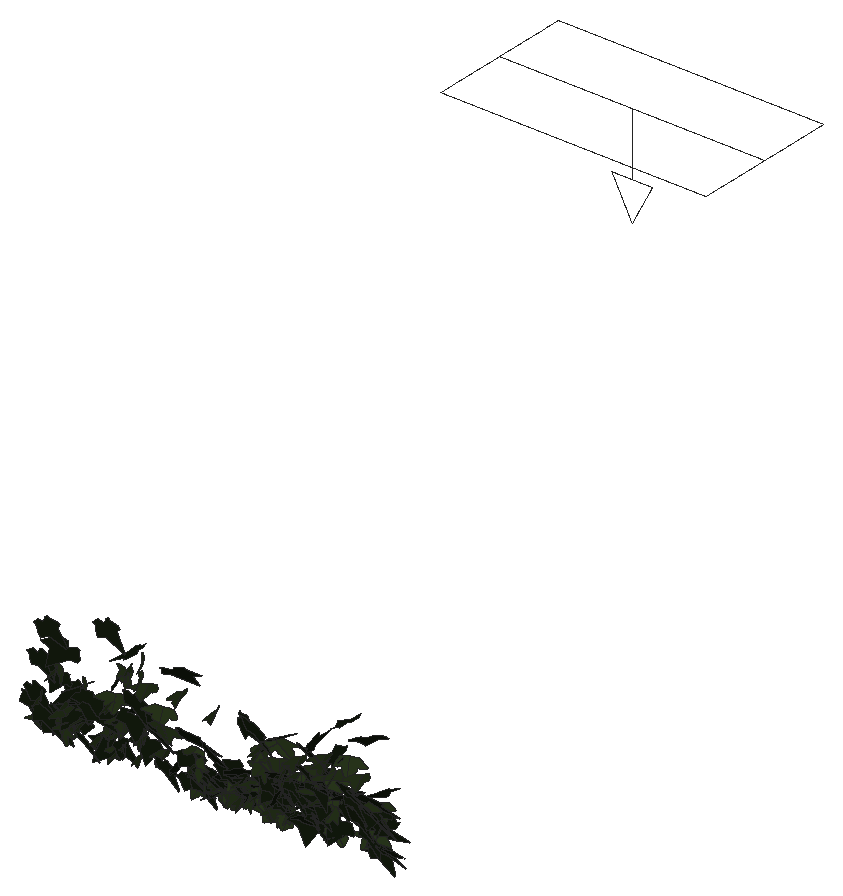
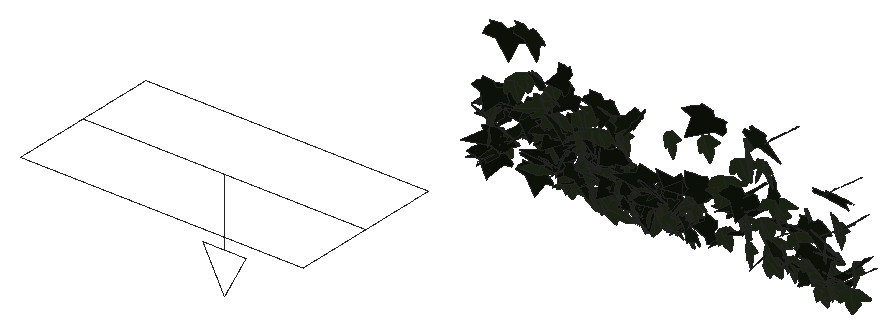
# SketchUp Ruby script. Lengths in millimetres.
U = 1.mm
M = Sketchup.active_model
def pt(a) = Geom::Point3d.new(a.map { |v| v * U })
def face(e, loops, mat)
  f = e.add_face(loops[0].map { |a| pt(a) })
  loops[1..].each { |l| e.add_face(l.map { |a| pt(a) }).erase! }
  f.material = f.back_material = mat if mat
  f
end
# faces: each face lists its corners as indices into pts; further lists are holes
def faces(e, pts, list, mat = nil) = list.each { |f| face(e, (f[0].is_a?(Array) ? f : [f]).map { |l| l.map { |i| pts[i] } }, mat) }
# xy, xz, yz: faces in a plane at the given z, y or x. An outline is a flat list of corners, or four numbers for a rectangle; further outlines are holes
def ring(l) = l.size == 4 ? [[l[0], l[1]], [l[2], l[1]], [l[2], l[3]], [l[0], l[3]]] : l.each_slice(2).to_a
def flat(e, list, mat, &to3) = list.each { |f| face(e, (f[0].is_a?(Array) ? f : [f]).map { |l| ring(l).map { |u, v| to3.(u, v) } }, mat) }
def xy(e, z, list, mat = nil) = flat(e, list, mat) { |x, y| [x, y, z] }
def xz(e, y, list, mat = nil) = flat(e, list, mat) { |x, z| [x, y, z] }
def yz(e, x, list, mat = nil) = flat(e, list, mat) { |y, z| [x, y, z] }
def lines(e, pts, list) = list.each { |a, b| e.add_line(pt(pts[a]), pt(pts[b])) }
# prism: a flat outline (further loops are holes) pulled along v
def prism(e, loops, v, mat = nil)
  f = face(e, loops, mat); d = Geom::Vector3d.new(v.map { |x| x * U })
  f.pushpull(f.normal.samedirection?(d) ? d.length : -d.length)
end
def box(e, o, s, mat = nil) = prism(e, [[o, [o[0] + s[0], o[1], o[2]], [o[0] + s[0], o[1] + s[1], o[2]], [o[0], o[1] + s[1], o[2]]]], [0, 0, s[2]], mat)
def at(x, y, z, deg = 0) = Geom::Transformation.translation(pt([x, y, z])) * Geom::Transformation.rotation(ORIGIN, Z_AXIS, deg.degrees)
def axes(o, x, y, z) = Geom::Transformation.new([*x, 0, *y, 0, *z, 0, *pt(o).to_a, 1])
def part(name) = M.definitions.add(name)
# library, detail: a bought-in or finely detailed component or shape, given as its bounding box
def library(name, o, s) = part(name).tap { |d| box(d.entities, o, s) }
def detail(e, o, s) = box(e.add_group.entities, o, s)
def put(e, d, t, mat = nil) = e.add_instance(d, t).tap { |i| i.material = mat if mat }
def group(e, t, mat = nil) = e.add_group.tap { |g| g.transformation = t; g.material = mat if mat }.entities
root = M.entities
M.materials.add("efeu1").color = [18, 25, 13]
M.materials.add("efeu2").color = [43, 57, 29]
c1 = part("ivyleaf_10")
p = [[0,12.8,-0.8],[-1.5,51.3,-10.9],[-4.9,51,-11.6],[-13.6,26.5,-7.3],[-13.2,15.9,-4.6],[-21.1,19.3,-7.2],
  [-29.5,16.3,-8.3],[-29.2,8.3,-6.2],[-19.7,-9.8,0.5],[-7.6,-13,4],[1,-12.2,5.8],[-0.4,51.1,-11.1],
  [-1.5,51.1,-10.9],[1,-12.4,5.9],[16.9,-12.4,3.5],[35.1,9.1,-5.1],[35,12.9,-6.1],[20.5,16.4,-4.9],
  [15.8,15,-3.8],[15.3,27.6,-7.1],[12.8,31.3,-7.8]]
faces(c1.entities,p,[[0,1,2,3,4,5,6,7,8,9,10],[11,12,0,13,14,15,16,17,18,19,20]],"efeu2")
c2 = part("ivyleaf_9")
p = [[39.1,54.8,31.7],[34.5,51.8,30.2],[-5.3,25.2,17.3],[-17.9,28.3,20.9],[-21.6,21.7,17],[-20.2,4.3,5.3],
  [-22.9,-0.3,2.5],[-17.1,-4,-0.6],[-2,-2.1,-1.2],[-0.7,-15.4,-10.1],[16.6,-22.3,-16.7],[21.1,-15.1,-12.5],
  [32.7,-10.7,-11],[46.1,-1.8,-6.6],[30.8,11.2,3.8]]
faces(c2.entities,p,[[0,1,2,3,4,5,6,7,8,9,10,11,12,13,14]],"efeu1")
c3 = part("Group240\#1")
p = [[0,0,0],[0,0,-197.7],[-63.2,0,-197.7],[411.6,-228.5,0],[-411.6,-228.5,0],[411.6,228.5,0],
  [411.6,0,0],[-411.6,228.5,0],[63.2,0,-197.7],[-411.6,0,0],[0,0,-320]]
lines(c3.entities,p,[[0,1],[1,2],[3,4],[5,6],[7,5],[1,8],[9,0],[0,6],[8,10],[4,9],[6,3],[2,10],
  [9,7]])
c4 = part("Rectangle Light\#2")
put(c4.entities,c3,at(0,0,0))
put(root,c1,axes([2467.9,943.6,1872.4],[-0.26486,-0.88516,0.00004],[-0.00622,0.00047,-0.89602],[1.68462,-0.13916,-0.0033]))
put(root,c1,axes([2705.5,950.2,1793.7],[0.91031,-0.25372,0.7536],[1.32752,-0.28837,-0.53979],[0.7266,0.84471,0.04208]))
put(root,c1,axes([2420.8,938.9,1761.7],[-1.66373,0.07531,0.0181],[-0.0341,0.00288,-0.87741],[-0.14341,-0.87436,-0.00133]))
put(root,c2,axes([2316.7,953.3,1750.5],[-0.39409,-0.85297,0.01207],[0.00655,-0.01326,-0.87772],[1.62353,-0.20699,0.00647]))
put(root,c1,axes([2361.1,945.6,1853.5],[-0.87128,-0.74486,0.14939],[-0.04243,-0.16117,-0.87192],[1.44522,-0.45378,0.06446]))
put(root,c2,axes([3038.7,936,1785.1],[1.61238,-0.09249,0.25483],[0.49062,0.01608,-0.85118],[0.15967,0.88454,0.04212]))
put(root,c1,axes([2910.3,944.7,1850.7],[-0.6012,-0.83319,0.06967],[0.02337,-0.07909,-0.89019],[1.59108,-0.31366,0.0394]))
put(root,c1,axes([2344,947.8,1718],[0.72212,-0.75077,0.22454],[0.4013,-0.14246,-0.83264],[1.43639,0.41724,0.11974]))
put(root,c1,axes([2796.7,947.1,1765.9],[0.88227,-0.70071,0.2164],[0.46375,-0.09429,-0.82731],[1.31643,0.50283,0.14642]))
put(root,c1,axes([2682.9,937.4,1657.3],[0.9527,-0.56773,-0.41231],[-0.3179,0.3955,-0.74738],[1.297,0.51396,0.11967]))
put(root,c2,axes([2330.5,942,1942.5],[-0.88006,0.71726,-0.27291],[0.03704,-0.30756,-0.84131],[-1.46009,-0.44013,0.14315]))
put(root,c1,axes([2261.2,947,1788.5],[-1.27395,-0.57202,0.12507],[0.12482,-0.26201,-0.84733],[1.10738,-0.62853,0.23939]))
put(root,c1,axes([3023,946,1834],[-0.68727,-0.80854,0.10452],[0.03048,-0.12133,-0.88322],[1.55132,-0.35582,0.06366]))
put(root,c2,axes([2679.9,953.4,1854.5],[0.65585,-0.85266,0.25567],[0.23139,-0.2265,-0.91927],[1.67828,0.36444,0.02683]))
put(root,c2,axes([3057.5,948.2,1747.2],[1.01963,-0.67289,0.13481],[0.14364,-0.11221,-0.86005],[1.29817,0.54093,-0.01072]))
put(root,c2,axes([2190,941.3,1740.7],[0.65041,-0.70724,-0.41439],[0.11605,0.46966,-0.75127],[1.55573,0.26064,0.22929]))
put(root,c2,axes([2769.1,930,1680.7],[0.1576,-0.22127,0.85612],[0.86263,0.74893,0.14972],[-1.445,0.42296,0.18276]))
put(root,c1,axes([2710.1,946,1801.6],[0.01408,-0.89116,0.03833],[-0.00107,-0.03834,-0.89119],[1.69763,0.00736,-0.00088]))
put(root,c2,axes([2231.7,945.4,1980.4],[0.44976,-0.80397,-0.30337],[-0.05454,0.30709,-0.83613],[1.63451,0.23147,0.05557]))
put(root,c2,axes([2549.8,939.8,1678],[1.3016,-0.47552,-0.21419],[-0.21038,0.21303,-0.8259],[0.97003,0.68426,0.10828]))
put(root,c2,axes([2756.8,959.4,1711.9],[-1.13486,-0.57406,0.25472],[0.02832,-0.36406,-0.78564],[1.19494,-0.53657,0.26053]))
put(root,c2,axes([2776.3,929,1862.9],[0.53766,0.81104,0.16092],[-0.04042,0.17712,-0.85538],[-1.57315,0.27264,0.07698]))
put(root,c2,axes([2596.5,941.1,1650.7],[-0.70916,0.74438,-0.22777],[0.13305,-0.2195,-0.83171],[-1.47555,-0.37755,0.03448]))
put(root,c2,axes([2817.1,952.6,1730],[0.17226,-0.85614,-0.00431],[-0.02833,0.00276,-0.86079],[1.62917,0.09057,-0.01451]))
put(root,c1,axes([2938.2,944.8,1811.7],[0.50976,-0.85015,-0.09039],[-0.00673,0.09362,-0.89101],[1.62712,0.26673,0.02463]))
put(root,c2,axes([2004.4,954.7,1693.1],[-0.03885,-0.85712,0.0673],[0.01629,-0.06752,-0.8573],[1.63621,-0.01968,0.01013]))
put(root,c2,axes([3004.6,952.1,1769],[0.19705,-0.87319,-0.05486],[0.00113,0.05531,-0.87928],[1.66514,0.1033,0.00709]))
put(root,c2,axes([2819.9,955.3,1756],[-0.70981,-0.79026,-0.03407],[0.06483,0.02158,-0.87358],[1.50402,-0.37389,0.02158]))
put(root,c1,axes([2780.2,943,1777.8],[0.86751,-0.73664,-0.18739],[-0.00785,0.2161,-0.85954],[1.44661,0.44293,0.10771]))
put(root,c1,axes([2109.7,939.1,1699.3],[-0.69981,-0.72469,-0.32601],[0.24848,0.29924,-0.81244],[1.49181,-0.3898,-0.01761]))
put(root,c2,axes([2048.8,947.2,1678.2],[-0.01924,-0.79231,-0.36591],[0.01801,0.36581,-0.79236],[1.66087,-0.01315,0.00435]))
put(root,c1,axes([2094.2,943.9,1646.4],[-1.33967,0.42463,-0.15601],[0.15741,-0.16289,-0.81655],[-0.84645,-0.70234,0.09506]))
put(root,c2,axes([2822.5,952.6,1746.8],[-0.02178,-0.87439,-0.09647],[-0.00803,0.09654,-0.87445],[1.67422,-0.01091,-0.00545]))
put(root,c2,axes([2107.4,953.8,1869.4],[-1.59187,-0.22783,-0.10408],[0.23043,-0.05016,-0.86323],[0.41731,-0.84138,0.07964]))
put(root,c1,axes([2353.6,946.1,1709.7],[0.03956,-0.8764,-0.02765],[-0.00239,0.02762,-0.87664],[1.66879,0.02082,-0.0006]))
put(root,c2,axes([2761.6,939.2,1748],[1.11776,-0.20498,0.58914],[1.17354,0.06847,-0.59087],[0.17944,0.82905,0.19446]))
put(root,c1,axes([2507.7,948,1683.9],[0.21064,-0.85815,0.05755],[0.02757,-0.05616,-0.86523],[1.63668,0.11139,0.00717]))
put(root,c2,axes([2498.8,940,1658.9],[0.41772,-0.58169,-0.59289],[0.01772,0.61492,-0.59986],[1.58068,0.14683,0.16341]))
put(root,c2,axes([3059.5,954.3,1764.8],[-1.26539,-0.50789,-0.24826],[0.46841,0.08498,-0.83298],[0.9686,-0.70461,0.07849]))
put(root,c2,axes([2884.2,925.3,1878.6],[0.2539,0.24727,0.91679],[0.89394,0.78742,-0.28073],[-1.57061,0.48815,-0.01157]))
put(root,c2,axes([2151.7,956.6,1635.3],[0.54439,-0.70731,0.40705],[0.27908,-0.37976,-0.76294],[1.52787,0.32139,-0.00567]))
put(root,c2,axes([2861.5,939.6,1853.5],[1.65475,-0.26156,-0.28108],[-0.51333,0.07912,-0.90794],[0.52006,0.91033,-0.00185]))
put(root,c1,axes([2737.8,942.1,1662.1],[-1.53367,0.31222,-0.04686],[0.08019,-0.02096,-0.8642],[-0.5955,-0.80693,0.00432]))
put(root,c2,axes([2022.3,950.1,1822.5],[0.45856,-0.83446,-0.16753],[-0.0346,0.16902,-0.86806],[1.61946,0.23989,0.02889]))
put(root,c2,axes([2193.8,956.4,1755.8],[-1.03123,-0.66738,-0.09407],[0.21794,0.02778,-0.85671],[1.26407,-0.54924,0.07097]))
put(root,c2,axes([2313.7,954.3,1803.7],[0.31449,-0.85872,0.01341],[-0.00061,-0.01372,-0.87447],[1.63451,0.16522,-0.00291]))
put(root,c2,axes([2363.2,951.9,1744.3],[0.9242,-0.70894,0.17463],[0.24251,-0.12422,-0.85862],[1.36826,0.50087,0.03423]))
put(root,c2,axes([2490.1,948.9,1706.7],[0.22463,-0.80548,-0.30843],[0.13705,0.31942,-0.80662],[1.6358,0.08385,0.10994]))
put(root,c2,axes([2594.9,950.3,1704.2],[0.80018,-0.76253,-0.03422],[0.08039,0.06225,-0.86818],[1.45048,0.41721,0.06699]))
put(root,c1,axes([2828.8,948.1,1814.3],[-0.46004,-0.85367,0.03783],[0.01161,-0.04104,-0.88707],[1.62626,-0.24119,0.01704]))
put(root,c2,axes([2701.3,934.4,1723.1],[0.15563,0.84621,0.05009],[-0.16196,0.05826,-0.84536],[-1.60517,0.07617,0.09015]))
put(root,c2,axes([2749.6,932.9,1826.6],[-0.04628,0.84008,0.20504],[-0.03955,0.20449,-0.84031],[-1.6453,-0.02854,0.01443]))
put(root,c1,axes([2712.6,943.5,1749.4],[1.19721,-0.54171,-0.29332],[-0.24451,0.29464,-0.81968],[1.14664,0.62843,0.13147]))
put(root,c1,axes([2913.3,948.2,1833.8],[-0.35011,-0.86827,0.02169],[0.00942,-0.02321,-0.8875],[1.65299,-0.18377,0.00965]))
put(root,c2,axes([2455.1,934.6,1936],[1.53035,0.42348,0.0933],[0.17778,0.02278,-0.90849],[-0.80591,0.80917,-0.02325]))
put(root,c2,axes([2882.3,956.2,1763.7],[0.09573,-0.87118,0.02439],[-0.00125,-0.02447,-0.87263],[1.65867,0.05026,-0.00207]))
put(root,c1,axes([2122.4,947.9,1661.6],[-0.72568,-0.78406,0.03692],[-0.02053,-0.03581,-0.87184],[1.49374,-0.3814,0.00595]))
put(root,c1,axes([2531.9,933.6,1692],[0.25909,-0.56883,-0.73164],[0.61868,0.72182,-0.50071],[1.65173,-0.18114,0.30232]))
put(root,c2,axes([2969,949.6,1787.5],[1.04021,-0.69755,0.00833],[0.15036,0.05138,-0.88119],[1.31913,0.5442,0.09387]))
put(root,c2,axes([2251.7,954.2,1651.2],[-1.58105,-0.14055,-0.11339],[0.21207,0.02113,-0.84254],[0.27048,-0.83817,-0.00222]))
put(root,c1,axes([2813.6,933.5,1696.6],[0.3828,0.06766,-0.86768],[-0.86684,0.76704,-0.04577],[1.41144,0.45273,0.20721]))
put(root,c1,axes([2881.7,951,1744.5],[-0.89868,-0.71255,0.14671],[-0.03727,-0.16239,-0.85174],[1.38406,-0.46703,0.07232]))
put(root,c1,axes([2404.3,954.1,1798.4],[-1.27482,-0.53387,0.18484],[0.12371,-0.35761,-0.79734],[1.0681,-0.59578,0.31296]))
put(root,c2,axes([2404.9,958,1649.7],[0.44725,-0.80998,0.18846],[0.10699,-0.17992,-0.84337],[1.57911,0.2416,0.00377]))
put(root,c2,axes([3030,954,1753.1],[0.93049,-0.7024,0.1556],[0.18839,-0.12067,-0.85572],[1.3562,0.49868,0.01211]))
put(root,c2,axes([2248.8,954.4,1745.2],[-1.61597,0.07599,0.12325],[-0.24749,-0.07772,-0.84791],[-0.1212,-0.85445,0.08809]))
put(root,c1,axes([2341.7,944.3,1868.8],[0.36417,-0.81308,-0.32498],[-0.0473,0.32747,-0.83395],[1.66582,0.18705,0.04737]))
put(root,c2,axes([2566.8,940.8,1685.1],[1.33692,-0.35338,-0.35224],[-0.3711,0.36548,-0.75552],[0.8741,0.69566,0.218]))
put(root,c2,axes([2537.4,961.6,1725.9],[0.31583,-0.40279,0.79125],[0.621,-0.72095,-0.43544],[1.57155,0.36583,0.01305]))
put(root,c1,axes([2091.7,944.7,1801.9],[0.86528,-0.68958,-0.30711],[-0.0766,0.33586,-0.81371],[1.43464,0.43384,0.14178]))
put(root,c2,axes([2077.1,964.5,1786],[-0.60418,-0.70125,0.37246],[-0.1548,-0.3703,-0.7665],[1.50324,-0.31998,0.07077]))
put(root,c1,axes([2298.4,940.7,1866.4],[0.73702,-0.53266,-0.59096],[-0.49411,0.53666,-0.65385],[1.43128,0.45956,0.07859]))
put(root,c2,axes([2737.8,954,1720.6],[0.33451,-0.83791,-0.15723],[0.00211,0.16076,-0.85548],[1.62253,0.17254,0.03353]))
put(root,c1,axes([2772,948.8,1788.6],[-1.3717,-0.4905,0.00951],[0.05881,-0.06226,-0.86908],[0.93183,-0.7181,0.06886]))
put(root,c2,axes([2658.5,942.8,1866.2],[0.96672,-0.53668,-0.55848],[-0.66997,0.43494,-0.73813],[1.31307,0.61704,0.03455]))
put(root,c2,axes([2998.9,955.6,1721],[0.70359,-0.78355,0.06825],[0.05768,-0.06116,-0.86639],[1.49579,0.37093,0.00131]))
put(root,c2,axes([2903.3,960.8,1728.6],[-0.84018,-0.74203,-0.00391],[0.09077,-0.02384,-0.86178],[1.40933,-0.44083,0.05318]))
put(root,c1,axes([2931.3,949.7,1708.6],[1.28701,-0.5645,-0.16398],[-0.19921,0.13032,-0.88029],[1.10088,0.68352,0.03241]))
put(root,c1,axes([2246.1,947.2,1764.7],[0.03971,-0.86574,-0.20459],[0.00101,0.20466,-0.86598],[1.69307,0.02018,0.00532]))
put(root,c1,axes([2886.8,942,1678.6],[-0.55208,0.77639,0.22455],[-0.21603,0.19708,-0.82802],[-1.52294,-0.3094,0.03605]))
put(root,c2,axes([3051,938,1956.8],[0.61842,0.83188,-0.10686],[-0.19135,-0.07514,-0.89066],[-1.58473,0.3337,0.06584]))
put(root,c2,axes([2840.1,949.9,1790.3],[1.22609,-0.60844,-0.01915],[0.14418,0.1078,-0.87649],[1.14955,0.63543,0.13035]))
put(root,c2,axes([2043.2,948.9,1917.1],[0.587,-0.72583,-0.40656],[-0.04612,0.42558,-0.77817],[1.58268,0.2816,0.12811]))
put(root,c1,axes([2986,949.9,1865.1],[1.11361,0.65554,-0.11344],[-0.26983,-0.02474,-0.87422],[-1.23708,0.59551,0.08856]))
put(root,c2,axes([2799.1,954.6,1705.5],[-1.53306,0.2288,-0.18474],[0.31242,-0.09712,-0.83604],[-0.46436,-0.8207,0.04743]))
put(root,c2,axes([2973.5,947.4,1734],[0.97047,-0.59501,-0.36846],[-0.39027,0.30886,-0.78254],[1.27351,0.54807,0.04097]))
put(root,c2,axes([2708.8,949.4,1669.3],[0.46911,0.5613,-0.58767],[-0.46184,-0.53525,-0.61302],[-1.47609,0.34585,0.00504]))
put(root,c1,axes([2766.4,944.3,1839.1],[1.29645,0.29451,0.46585],[0.6213,0.38113,-0.7183],[-0.84513,0.73197,0.18657]))
put(root,c1,axes([2170,943.7,1788],[0.43763,-0.69637,-0.47194],[-0.08556,0.47838,-0.72777],[1.59872,0.21622,0.09024]))
put(root,c1,axes([2237.6,949.9,1678.2],[0.73526,-0.74565,-0.13769],[0.17887,0.20043,-0.8217],[1.43198,0.35782,0.17334]))
put(root,c2,axes([2516.2,957,1641.9],[0.47088,-0.81913,-0.07357],[0.0296,0.08147,-0.85483],[1.56497,0.24493,0.0383]))
put(root,c1,axes([2694.9,955.2,1691.8],[1.42292,-0.37077,0.24795],[0.47448,-0.05394,-0.83239],[0.70392,0.78584,0.05985]))
put(root,c1,axes([2613.4,950.7,1636.5],[-1.40709,-0.37225,0.10008],[-0.1704,-0.04472,-0.82775],[0.71355,-0.74473,-0.00032]))
put(root,c1,axes([2821.1,955.1,1765.1],[-0.12246,-0.8658,0.10447],[-0.05796,-0.10246,-0.86789],[1.65872,-0.0675,-0.02261]))
put(root,c1,axes([2904.6,953.8,1783.9],[-0.7516,-0.78033,0.06766],[0.05443,-0.09009,-0.87207],[1.48969,-0.39041,0.066]))
put(root,c1,axes([2515.6,953.7,1630.9],[1.24501,-0.54678,-0.05877],[-0.07865,0.04219,-0.85257],[1.04367,0.65544,0.00585]))
put(root,c1,axes([3077.8,950.7,1770.8],[-1.25736,-0.5489,-0.16054],[0.38831,0.00292,-0.84964],[1.01681,-0.67987,0.12596]))
put(root,c2,axes([2986.9,937.7,1975.5],[0.01006,0.86938,0.22364],[-0.14922,0.22324,-0.86596],[-1.70194,-0.01443,0.07724]))
put(root,c2,axes([2867.7,942.4,1667.5],[0.98909,0.64386,-0.22357],[-0.34715,-0.1395,-0.82577],[-1.24985,0.54828,0.05243]))
put(root,c2,axes([2959.5,949.3,1871.5],[-1.08075,0.67413,-0.07436],[0.06867,-0.06682,-0.88129],[-1.28896,-0.56879,0.01539]))
put(root,c1,axes([2787.8,947,1772.8],[0.20165,-0.78561,-0.3752],[-0.0369,0.37575,-0.79222],[1.65653,0.104,0.02802]))
put(root,c1,axes([2566.3,951.4,1852.2],[-0.05275,-0.87059,-0.14113],[-0.00528,0.14129,-0.871],[1.67852,-0.02691,-0.00718]))
put(root,c1,axes([2284.7,952.9,1729.5],[-0.98379,-0.71114,-0.02205],[0.11719,-0.01756,-0.8771],[1.34901,-0.51708,0.06011]))
put(root,c2,axes([2895.5,943.6,1754.8],[0.99429,0.59745,-0.33857],[-0.59781,-0.1704,-0.78538],[-1.16222,0.59877,0.11432]))
put(root,c2,axes([2137.9,962.5,1702.6],[-1.4103,-0.42406,-0.03234],[0.05068,0.01856,-0.85377],[0.80782,-0.74149,-0.00288]))
put(root,c2,axes([2002.4,954.8,1721.6],[0.66275,-0.76295,-0.24811],[-0.10483,0.2471,-0.83715],[1.52328,0.34895,0.05033]))
put(root,c2,axes([2627.9,940.5,1706.9],[0.80073,-0.02688,0.7568],[1.28025,0.41088,-0.35937],[-0.66192,0.76219,0.22043]))
put(root,c1,axes([2497.2,962.1,1712.1],[0.50292,0.58423,-0.62362],[-0.712,-0.50779,-0.63424],[-1.46222,0.4482,0.09434]))
put(root,c2,axes([2866.2,962.2,1671.4],[0.34879,-0.84035,0.05099],[-0.0033,-0.05256,-0.86001],[1.6023,0.18282,-0.01287]))
put(root,c1,axes([2774.5,950.3,1738.4],[-0.74948,0.77477,0.0623],[-0.36984,-0.03052,-0.84884],[-1.43232,-0.39752,0.18658]))
put(root,c2,axes([2759.6,949,1710.1],[1.59715,-0.16882,0.03563],[0.06069,-0.02215,-0.85586],[0.32271,0.83965,-0.01541]))
put(root,c1,axes([2188.1,958.1,1726.4],[-0.75727,-0.75041,0.18218],[0.02116,-0.21049,-0.84273],[1.46951,-0.38367,0.10602]))
put(root,c1,axes([2262.7,962.2,1637.8],[-0.24892,-0.75175,0.3805],[-0.08078,-0.37869,-0.76276],[1.60153,-0.13594,0.02067]))
put(root,c2,axes([2352.8,967,1689.5],[-0.58891,-0.78496,0.11855],[0.01763,-0.1308,-0.84188],[1.51077,-0.30446,0.05603]))
put(root,c1,axes([2832,954.7,1759.3],[1.48089,0.40461,0.02343],[0.03195,0.01849,-0.87698],[-0.77068,0.77824,0.00866]))
put(root,c2,axes([2846,966.2,1642],[-0.63565,-0.78503,0.02418],[0.05186,-0.03785,-0.85219],[1.49387,-0.33272,0.03988]))
put(root,c1,axes([2642.2,966.2,1684.1],[-0.74241,-0.47484,0.59059],[-0.22658,-0.6176,-0.57518],[1.42435,-0.34574,0.21633]))
put(root,c2,axes([2868.6,957.3,1703.3],[0.46618,-0.78538,-0.25499],[-0.05531,0.2576,-0.82136],[1.57057,0.24219,0.04676]))
put(root,c1,axes([2025,949.2,1703.4],[0.08591,-0.78293,-0.37668],[0.11766,0.37913,-0.78061],[1.64937,0.01374,0.0753]))
put(root,c1,axes([2068.1,953.2,1790.5],[0.07515,-0.84868,-0.1854],[0.06464,0.18696,-0.84858],[1.65204,0.03129,0.04163]))
put(root,c1,axes([2650.4,957.4,1685],[-0.14758,-0.84578,0.03604],[-0.01332,-0.03555,-0.84932],[1.6111,-0.07777,-0.00372]))
put(root,c1,axes([2283.1,958.9,1718.8],[0.9157,-0.71154,0.07292],[0.15214,-0.03383,-0.85765],[1.35276,0.48545,0.0471]))
put(root,c1,axes([2107.9,953.5,1719.8],[0.1026,-0.82425,-0.20479],[0.05404,0.20683,-0.82501],[1.6155,0.04543,0.0406]))
put(root,c1,axes([2900.5,955.8,1723],[-0.40665,-0.8455,-0.05609],[0.04161,0.05233,-0.87204],[1.61216,-0.21462,0.00836]))
put(root,c2,axes([3039.5,965.9,1680.7],[0.15196,-0.84584,0.09159],[-0.01234,-0.0926,-0.84946],[1.61916,0.07868,-0.01507]))
put(root,c1,axes([2208.9,956.5,1654.5],[-0.02567,-0.86483,-0.06485],[0.01894,0.0647,-0.86489],[1.65045,-0.01419,0.00892]))
put(root,c1,axes([2603.8,966.7,1642.2],[-0.2302,-0.68836,0.4772],[0.32357,-0.49229,-0.66703],[1.56091,0.00053,0.20865]))
put(root,c2,axes([2587.3,940.9,1679.9],[1.07226,0.25057,0.59872],[0.91294,0.37331,-0.60762],[-0.8321,0.73248,0.10486]))
put(root,c2,axes([2139.4,959.4,1756.4],[-1.49804,0.32185,-0.13002],[0.21007,-0.07345,-0.84998],[-0.62635,-0.7944,0.02591]))
put(root,c2,axes([2767,959.9,1678.2],[0.34726,-0.80067,-0.25157],[0.0127,0.25883,-0.81891],[1.59723,0.17202,0.06121]))
put(root,c2,axes([2636.9,959.4,1708.9],[-1.51427,0.28436,-0.02191],[0.02531,-0.02785,-0.84465],[-0.54221,-0.79546,0.02175]))
put(root,c1,axes([2805.3,961.5,1712.6],[0.87746,-0.71773,0.13539],[0.20011,-0.09321,-0.85222],[1.37559,0.47139,0.03762]))
put(root,c2,axes([2060,954.9,1652.6],[0.2213,-0.67687,-0.5282],[0.03448,0.53484,-0.68139],[1.63368,0.0804,0.08593]))
put(root,c1,axes([2275.4,954.6,1646.1],[-0.05824,-0.83738,-0.23344],[0.00829,0.23343,-0.83793],[1.65445,-0.03064,-0.00402]))
put(root,c2,axes([2351.7,958.8,1758.4],[0.86776,-0.72125,-0.16298],[0.01203,0.19526,-0.84646],[1.40724,0.44308,0.10773]))
put(root,c2,axes([2870.9,947.1,1683.5],[0.90823,-0.00913,0.77376],[1.43221,0.21722,-0.46156],[-0.34303,0.88275,0.12158]))
put(root,c1,axes([3054.6,960,1676.9],[1.4009,0.34389,-0.30202],[-0.55886,-0.08389,-0.81118],[-0.66815,0.79119,0.04526]))
put(root,c1,axes([2540.8,961.7,1657.1],[-1.13091,-0.60841,0.14157],[0.06333,-0.22595,-0.83135],[1.18718,-0.56752,0.17921]))
put(root,c1,axes([2877.6,956.2,1789.1],[1.21378,-0.52621,-0.27544],[-0.29793,0.24094,-0.82277],[1.09042,0.65158,0.0818]))
put(root,c2,axes([2946.5,965.3,1673.5],[-1.47061,-0.20546,-0.31245],[0.58853,0.05222,-0.7991],[0.40018,-0.83184,0.02701]))
put(root,c2,axes([2464.5,955.6,1755.8],[1.54316,-0.25843,0.35026],[0.64564,-0.08882,-0.85084],[0.51906,0.87877,0.01701]))
put(root,c1,axes([2707.1,964.1,1691],[0.47193,-0.79606,0.19306],[0.27043,-0.15685,-0.82926],[1.53534,0.27232,0.08673]))
put(root,c1,axes([2575.6,962.9,1656.3],[-0.09348,-0.8447,0.12551],[-0.05488,-0.12401,-0.84585],[1.62435,-0.0528,-0.02135]))
put(root,c2,axes([2877,945.7,1762.3],[1.34216,0.52338,0.11083],[0.15554,0.07583,-0.87812],[-1.00623,0.70983,0.01209]))
put(root,c1,axes([2330.3,956.9,1645.6],[0.14724,-0.82771,-0.20258],[0.07415,0.20663,-0.8294],[1.62009,0.06577,0.05637]))
put(root,c1,axes([2643.9,962.6,1633.9],[0.04653,-0.84633,0.0904],[0.02318,-0.09008,-0.84663],[1.61974,0.0256,0.00952]))
put(root,c1,axes([2341,952.3,1914.2],[0.3119,-0.73005,-0.46171],[-0.07433,0.4632,-0.74628],[1.6423,0.15962,0.05391]))
put(root,c2,axes([2975.4,947.1,1765.8],[0.45263,0.83183,0.02298],[-0.0045,0.02458,-0.86511],[-1.58374,0.23766,0.00903]))
put(root,c1,axes([2687.7,961.6,1693.5],[-0.64019,-0.78053,0.07618],[-0.03743,-0.07447,-0.84985],[1.4921,-0.33676,0.01137]))
put(root,c1,axes([2251.3,960.2,1688.3],[-0.60999,-0.80189,-0.0093],[0.00138,0.00973,-0.86356],[1.52626,-0.32049,-0.00293]))
put(root,c1,axes([2940.5,942.7,1795],[0.02325,-0.03147,0.96719],[0.63208,0.90866,0.02537],[-1.72987,0.33159,0.02227]))
put(root,c1,axes([2817.3,954.1,1726.9],[-0.63088,0.80212,0.11016],[-0.10997,0.09529,-0.86775],[-1.53699,-0.33606,0.01687]))
put(root,c1,axes([2496.4,955.3,1699],[1.07537,-0.5662,-0.32944],[-0.16746,0.36552,-0.77912],[1.23542,0.54239,0.18115]))
put(root,c1,axes([2923.9,960.4,1729.2],[1.37542,0.46259,-0.0301],[-0.05157,-0.01349,-0.85806],[-0.88076,0.72319,0.00324]))
put(root,c2,axes([3107.2,949.6,1719.1],[-0.59763,0.55915,0.59705],[-0.77323,0.44846,-0.63367],[-1.35121,-0.50394,0.09855]))
put(root,c1,axes([2623.7,962.3,1636.6],[-1.06687,-0.6392,0.08068],[0.05206,-0.13046,-0.84354],[1.22508,-0.55111,0.1061]))
put(root,c1,axes([2303.2,943.1,1862.8],[-0.02006,0.17131,0.86807],[-0.69357,0.79024,-0.16038],[-1.53451,-0.35941,0.06114]))
put(root,c1,axes([2143.3,963.8,1663],[0.22259,-0.83454,0.06646],[0.00638,-0.06664,-0.84267],[1.59331,0.11685,-0.00591]))
put(root,c1,axes([2649.4,963.9,1649.9],[0.76106,-0.74958,0.06657],[0.14328,-0.03516,-0.84812],[1.42504,0.40386,0.04972]))
put(root,c1,axes([2664.9,958.3,1660],[0.66329,-0.73884,-0.28075],[-0.2326,0.25277,-0.81691],[1.48617,0.36931,-0.00255]))
put(root,c2,axes([2270.7,954.9,1660.5],[0.69685,-0.5321,-0.55869],[-0.52977,0.48566,-0.64497],[1.36949,0.45862,0.03479]))
put(root,c1,axes([2747.9,961.8,1641.7],[-0.42022,-0.83333,-0.00911],[0.02452,0.00601,-0.86201],[1.5859,-0.2209,0.01091]))
put(root,c1,axes([2697,963.9,1664.3],[0.15358,-0.85466,0.02079],[-0.0156,-0.02165,-0.8584],[1.627,0.08047,-0.01019]))
put(root,c2,axes([2884.7,955.9,1769.8],[1.45363,-0.42176,-0.05989],[0.19405,0.30037,-0.81499],[0.78717,0.70479,0.3115]))
put(root,c2,axes([2719.6,961.8,1738.8],[-0.10552,-0.04098,0.85432],[1.4783,-0.36081,0.0331],[0.68146,0.77637,0.06048]))
put(root,c1,axes([2847.4,965.1,1648.5],[-0.93429,-0.69208,0.11224],[0.04029,-0.15159,-0.8421],[1.33376,-0.48022,0.10406]))
put(root,c1,axes([2590.5,959.8,1662.8],[-1.4932,0.16122,0.32304],[-0.64259,-0.05396,-0.79309],[-0.24335,-0.84676,0.11204]))
put(root,c1,axes([2662.9,964.2,1663.9],[0.12411,-0.85643,-0.01203],[-0.00264,0.01196,-0.85891],[1.63012,0.06523,-0.00048]))
put(root,c1,axes([2173.8,960.5,1711.6],[0.41103,-0.80844,-0.22185],[-0.02374,0.22596,-0.83559],[1.59533,0.21166,0.04472]))
put(root,c2,axes([2144.8,951.4,1775.7],[0.09793,0.85892,0.02038],[-0.14301,0.02483,-0.85706],[-1.6289,0.04946,0.07647]))
put(root,c1,axes([2151.6,963.9,1679.3],[-0.30907,-0.84302,-0.01114],[-0.03412,0.0148,-0.85828],[1.60422,-0.1621,-0.0204]))
put(root,c1,axes([3081.2,954.5,1741.8],[-0.95975,0.65155,0.2966],[-0.33149,0.24023,-0.82386],[-1.32152,-0.53344,-0.00875]))
put(root,c2,axes([2443.3,947.4,1650.1],[0.31124,0.01722,0.84757],[0.89266,0.71721,-0.10507],[-1.34399,0.48035,0.12649]))
put(root,c2,axes([2492.5,971.3,1658.1],[0.48512,-0.8035,0.04285],[0.01206,-0.04294,-0.84293],[1.53134,0.25488,-0.00694]))
put(root,c2,axes([2100.6,968.7,1668.7],[-1.53411,0.22484,0.13716],[-0.33116,-0.1231,-0.82078],[-0.37628,-0.80834,0.16315]))
put(root,c1,axes([2780.8,966.7,1634.2],[1.59074,-0.05974,-0.04926],[-0.0942,-0.00152,-0.83794],[0.11333,0.83727,-0.00503]))
put(root,c1,axes([2394.4,970.4,1670.5],[-0.27822,-0.80825,0.19938],[-0.01887,-0.20073,-0.82098],[1.58426,-0.14433,0.02523]))
put(root,c2,axes([2166.2,963.4,1679.1],[-1.30325,0.49699,0.06428],[-0.08672,0.04664,-0.84605],[-0.94981,-0.6862,-0.01095]))
put(root,c2,axes([2252,962.4,1690.1],[-0.74567,0.73601,-0.2047],[0.18875,-0.1791,-0.83378],[-1.44163,-0.40414,-0.00329]))
put(root,c2,axes([2260.7,947.6,1822.4],[0.09816,0.32593,0.81256],[0.37428,0.78885,-0.32891],[-1.62365,0.20155,-0.0267]))
put(root,c1,axes([2638.6,968.6,1635.8],[0.19519,-0.84329,-0.00153],[0.0042,0.00181,-0.8495],[1.60494,0.10256,0.00241]))
put(root,c2,axes([3062.6,969.7,1641.3],[0.29748,-0.78722,-0.26729],[-0.04737,0.26742,-0.80216],[1.58154,0.15608,0.02625]))
put(root,c1,axes([2766.2,970,1634.8],[1.2337,-0.5421,0.01637],[0.0233,-0.01088,-0.84502],[1.03192,0.64834,-0.00049]))
put(root,c1,axes([2115.5,962.6,1675.7],[-0.97178,-0.61685,-0.28483],[0.3661,0.21048,-0.80065],[1.24019,-0.54548,0.01316]))
put(root,c1,axes([2090.1,964.6,1660],[0.13864,-0.81952,-0.23105],[-0.02566,0.23075,-0.82272],[1.6203,0.07378,0.00674]))
put(root,c2,axes([2827.2,957.7,1679.1],[-0.04134,0.85905,-0.06341],[-0.01618,-0.06364,-0.85927],[-1.63932,-0.02103,0.01008]))
put(root,c2,axes([2345.1,954.7,1780.7],[0.93641,0.72434,-0.01563],[-0.04785,-0.00181,-0.87542],[-1.37805,0.49226,0.01978]))
put(root,c1,axes([2774.8,964.6,1704.9],[-1.59804,-0.17869,-0.05465],[0.10085,0.01358,-0.85846],[0.34103,-0.84133,-0.00224]))
put(root,c2,axes([2665.9,959.2,1693.6],[0.74726,0.67621,-0.34872],[-0.60468,-0.21084,-0.76657],[-1.31572,0.48095,0.15425]))
put(root,c1,axes([2701.8,968.1,1665.7],[1.60104,0.35034,0.16637],[0.29005,0.06679,-0.91126],[-0.67875,0.85492,0.00302]))
put(root,c2,axes([2712.5,956.6,1694.6],[1.31707,0.50832,0.0779],[0.14054,0.03102,-0.85846],[-0.96859,0.69571,-0.01864]))
put(root,c2,axes([3073.2,953.2,1803.8],[0.68918,0.75936,0.24923],[0.18032,0.2309,-0.84118],[-1.51034,0.37407,0.0133]))
put(root,c1,axes([2333.2,967.2,1705.2],[0.80381,-0.71185,-0.2197],[-0.04523,0.23955,-0.82185],[1.41713,0.41142,0.09839]))
put(root,c1,axes([2022.3,969.4,1642.4],[-0.9623,-0.66715,0.00749],[0.00836,-0.01273,-0.83703],[1.26977,-0.50551,0.01119]))
put(root,c1,axes([2931.9,966.6,1650.3],[1.02371,0.64418,0.14873],[0.19427,0.10851,-0.83917],[-1.24316,0.54742,-0.00867]))
put(root,c2,axes([3070.5,960,1640.8],[1.20477,0.53677,-0.22177],[-0.41211,-0.08626,-0.82686],[-1.02565,0.66518,0.07174]))
put(root,c1,axes([2068.3,978.2,1646.6],[0.10159,-0.76144,0.32186],[0.14126,-0.31681,-0.76181],[1.56697,0.07793,0.04781]))
put(root,c2,axes([2639.6,965.5,1665.1],[0.75353,0.59622,-0.46108],[-0.53746,-0.36554,-0.71517],[-1.32996,0.48553,0.02777]))
put(root,c2,axes([3056.2,970.9,1652.2],[1.09336,-0.61904,-0.04635],[0.14245,0.13177,-0.83212],[1.17284,0.56109,0.14428]))
put(root,c1,axes([3076.7,963.9,1708],[0.22378,-0.72401,-0.44865],[0.13076,0.45949,-0.7235],[1.61577,0.06309,0.12069]))
put(root,c1,axes([2735.4,962.2,1689.3],[-0.2815,-0.09482,0.84424],[1.22119,0.54917,0.17409],[-1.05969,0.65805,-0.02364]))
put(root,c1,axes([2707.3,969.7,1645.5],[0.52255,-0.04166,-0.80063],[1.51961,-0.0621,0.27705],[-0.13758,-0.84412,0.01913]))
put(root,c1,axes([2602,967.6,1640.4],[-1.53981,0.15739,0.19616],[-0.3612,0.05153,-0.82411],[-0.31407,-0.83091,-0.01395]))
put(root,c2,axes([2888.8,954.6,1774.9],[0.15457,0.58589,0.6476],[-0.26347,0.65081,-0.57143],[-1.64106,-0.0493,0.15274]))
put(root,c2,axes([2127.8,964.9,1718.3],[0.46323,0.77377,-0.27334],[-0.40775,-0.2153,-0.80026],[-1.50766,0.29597,0.13245]))
put(root,c2,axes([3047.9,960.9,1691.3],[0.12484,0.16208,-0.84665],[0.60748,0.78418,0.17485],[1.52399,-0.32586,-0.00034]))
put(root,c1,axes([2102.4,980,1630.9],[-0.19661,-0.79687,0.19354],[0.0041,-0.19533,-0.8031],[1.56068,-0.09987,0.02649]))
put(root,c2,axes([2945.2,960.2,1636],[0.52235,0.78455,0.18613],[-0.09073,0.21206,-0.82356],[-1.53192,0.25496,0.11224]))
put(root,c1,axes([2726.9,970.8,1619.7],[0.04252,-0.02076,-0.95461],[-1.59296,0.45911,-0.02957],[0.87456,0.83726,-0.00745]))
put(root,c1,axes([2065.7,967.5,1635.2],[0.70729,0.21744,-0.72133],[1.13942,0.40303,0.42994],[0.87042,-0.70427,0.02333]))
put(root,c1,axes([2674.6,968.5,1654.2],[0.80823,-0.33661,0.74541],[-1.14645,0.4394,0.54161],[-1.05292,-0.73682,-0.01754]))
put(root,c2,axes([2489.7,968,1647.7],[0.25633,0.46315,0.75382],[0.09652,0.7572,-0.4743],[-1.68105,0.1141,0.08771]))
put(root,c4,at(2371.7,2815.1,2644.1,180))
